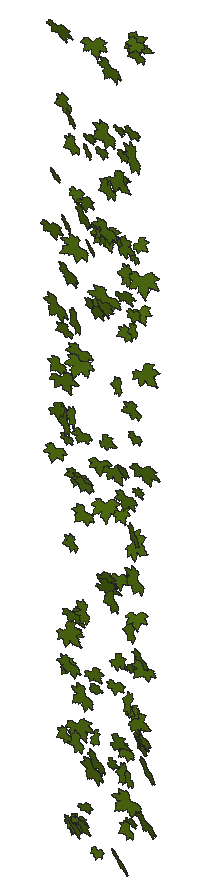
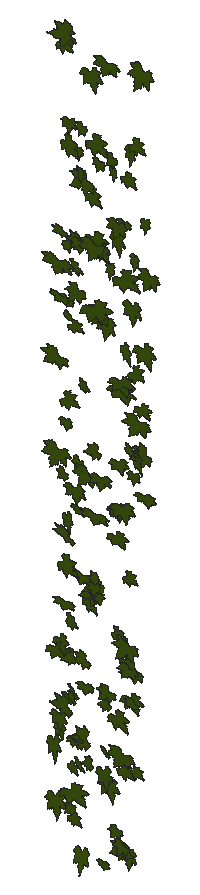
# SketchUp Ruby script. Lengths in inches.
U = 1.inch
M = Sketchup.active_model
def pt(a) = Geom::Point3d.new(a.map { |v| v * U })
def face(e, loops, mat)
  f = e.add_face(loops[0].map { |a| pt(a) })
  loops[1..].each { |l| e.add_face(l.map { |a| pt(a) }).erase! }
  f.material = f.back_material = mat if mat
  f
end
# faces: each face lists its corners as indices into pts; further lists are holes
def faces(e, pts, list, mat = nil) = list.each { |f| face(e, (f[0].is_a?(Array) ? f : [f]).map { |l| l.map { |i| pts[i] } }, mat) }
# xy, xz, yz: faces in a plane at the given z, y or x. An outline is a flat list of corners, or four numbers for a rectangle; further outlines are holes
def ring(l) = l.size == 4 ? [[l[0], l[1]], [l[2], l[1]], [l[2], l[3]], [l[0], l[3]]] : l.each_slice(2).to_a
def flat(e, list, mat, &to3) = list.each { |f| face(e, (f[0].is_a?(Array) ? f : [f]).map { |l| ring(l).map { |u, v| to3.(u, v) } }, mat) }
def xy(e, z, list, mat = nil) = flat(e, list, mat) { |x, y| [x, y, z] }
def xz(e, y, list, mat = nil) = flat(e, list, mat) { |x, z| [x, y, z] }
def yz(e, x, list, mat = nil) = flat(e, list, mat) { |y, z| [x, y, z] }
def lines(e, pts, list) = list.each { |a, b| e.add_line(pt(pts[a]), pt(pts[b])) }
# prism: a flat outline (further loops are holes) pulled along v
def prism(e, loops, v, mat = nil)
  f = face(e, loops, mat); d = Geom::Vector3d.new(v.map { |x| x * U })
  f.pushpull(f.normal.samedirection?(d) ? d.length : -d.length)
end
def box(e, o, s, mat = nil) = prism(e, [[o, [o[0] + s[0], o[1], o[2]], [o[0] + s[0], o[1] + s[1], o[2]], [o[0], o[1] + s[1], o[2]]]], [0, 0, s[2]], mat)
def at(x, y, z, deg = 0) = Geom::Transformation.translation(pt([x, y, z])) * Geom::Transformation.rotation(ORIGIN, Z_AXIS, deg.degrees)
def axes(o, x, y, z) = Geom::Transformation.new([*x, 0, *y, 0, *z, 0, *pt(o).to_a, 1])
def part(name) = M.definitions.add(name)
# library, detail: a bought-in or finely detailed component or shape, given as its bounding box
def library(name, o, s) = part(name).tap { |d| box(d.entities, o, s) }
def detail(e, o, s) = box(e.add_group.entities, o, s)
def put(e, d, t, mat = nil) = e.add_instance(d, t).tap { |i| i.material = mat if mat }
def group(e, t, mat = nil) = e.add_group.tap { |g| g.transformation = t; g.material = mat if mat }.entities
root = M.entities
M.materials.add("[Vegetation Blur 03]").color = [83, 114, 18]
c1 = part("ivy")
xy(c1.entities,0,[[0.782,0,0.786,0,0.787,0.005,0.789,0.009,0.821,0.072,0.875,0.147,1.001,0.272,1.073,0.331,1.137,0.363,1.178,0.379,1.223,0.384,1.272,0.383,1.311,0.374,1.36,0.355,1.399,0.334,1.491,0.285,1.541,0.244,1.583,0.199,1.617,0.15,1.64,0.128,1.662,0.115,1.717,0.105,1.745,0.093,1.784,0.054,1.819,0.057,1.854,0.064,1.882,0.075,1.896,0.074,1.91,0.071,1.937,0.063,1.964,0.053,1.99,0.038,2.016,0.015,2.034,0.002,2.04,0,2.038,0.003,2.036,0.007,2.033,0.038,2.036,0.068,2.045,0.1,2.055,0.116,2.064,0.123,2.077,0.129,2.088,0.129,2.106,0.132,2.118,0.13,2.179,0.132,2.207,0.133,2.225,0.133,2.242,0.138,2.22,0.162,2.207,0.186,2.206,0.213,2.212,0.236,2.228,0.262,2.247,0.274,2.298,0.283,2.355,0.294,2.37,0.296,2.376,0.295,2.377,0.3,2.377,0.303,2.385,0.329,2.411,0.37,2.426,0.392,2.449,0.407,2.511,0.426,2.561,0.444,2.619,0.466,2.589,0.469,2.561,0.476,2.501,0.5,2.449,0.516,2.424,0.523,2.401,0.535,2.377,0.556,2.372,0.568,2.36,0.575,2.268,0.586,2.225,0.592,2.207,0.599,2.194,0.61,2.143,0.65,2.13,0.664,2.122,0.682,2.123,0.7,2.13,0.719,2.148,0.75,2.17,0.781,2.195,0.807,2.221,0.828,2.284,0.874,2.291,0.88,2.288,0.887,2.276,0.9,2.267,0.916,2.265,0.933,2.273,0.967,2.292,1.002,2.313,1.03,2.334,1.054,2.348,1.067,2.358,1.074,2.363,1.076,2.362,1.081,2.35,1.094,2.347,1.11,2.35,1.143,2.359,1.18,2.385,1.254,2.415,1.324,2.448,1.393,2.45,1.4,2.446,1.398,2.44,1.394,2.427,1.383,2.402,1.36,2.376,1.339,2.345,1.324,2.305,1.309,2.282,1.303,2.273,1.306,2.245,1.294,2.212,1.287,2.187,1.291,2.163,1.301,2.142,1.316,2.134,1.327,2.124,1.325,2.09,1.292,2.053,1.259,2.014,1.234,1.973,1.215,1.954,1.21,1.931,1.208,1.909,1.212,1.893,1.22,1.879,1.233,1.872,1.248,1.867,1.281,1.864,1.319,1.821,1.258,1.773,1.197,1.726,1.141,1.698,1.121,1.679,1.116,1.666,1.117,1.647,1.122,1.632,1.129,1.62,1.141,1.617,1.154,1.617,1.219,1.621,1.254,1.623,1.268,1.623,1.281,1.618,1.314,1.606,1.346,1.603,1.375,1.607,1.403,1.603,1.467,1.599,1.499,1.605,1.525,1.614,1.552,1.629,1.577,1.635,1.589,1.629,1.587,1.618,1.582,1.596,1.566,1.581,1.556,1.568,1.552,1.557,1.55,1.545,1.553,1.531,1.562,1.522,1.572,1.504,1.591,1.486,1.611,1.474,1.631,1.457,1.666,1.455,1.684,1.457,1.698,1.452,1.715,1.444,1.728,1.424,1.754,1.419,1.772,1.423,1.786,1.434,1.819,1.444,1.848,1.446,1.855,1.44,1.861,1.43,1.867,1.386,1.904,1.349,1.948,1.326,1.973,1.31,1.995,1.288,2.048,1.284,2.153,1.287,2.254,1.284,2.255,1.282,2.253,1.278,2.247,1.274,2.237,1.266,2.216,1.226,2.125,1.208,2.076,1.184,2.033,1.155,1.984,1.135,1.942,1.111,1.899,1.083,1.861,1.053,1.85,1.059,1.83,1.061,1.809,1.056,1.79,1.049,1.767,1.04,1.749,1.018,1.733,0.994,1.726,0.942,1.734,0.95,1.6875,0.944,1.645,0.932,1.608,0.911,1.585,0.881,1.58,0.854,1.582,0.828,1.588,0.785,1.618,0.773,1.625,0.775,1.614,0.779,1.598,0.796,1.502,0.818,1.402,0.861,1.283,0.882,1.224,0.894,1.174,0.892,1.148,0.886,1.123,0.881,1.107,0.872,1.099,0.849,1.094,0.818,1.092,0.789,1.098,0.762,1.107,0.753,1.113,0.721,1.139,0.698,1.163,0.678,1.194,0.665,1.224,0.628,1.28,0.612,1.312,0.606,1.327,0.606,1.314,0.599,1.282,0.594,1.267,0.581,1.256,0.544,1.245,0.512,1.244,0.473,1.249,0.444,1.256,0.382,1.288,0.339,1.306,0.324,1.316,0.317,1.324,0.309,1.326,0.27,1.314,0.227,1.313,0.185,1.3125,0.152,1.317,0.122,1.328,0.092,1.345,0.073,1.353,0.079,1.338,0.092,1.308,0.117,1.249,0.13,1.215,0.139,1.164,0.147,1.148,0.157,1.136,0.163,1.122,0.174,1.086,0.177,1.067,0.182,1.054,0.186,1.043,0.191,1.038,0.211,1.028,0.237,1.005,0.25,0.974,0.253,0.96,0.25,0.944,0.242,0.914,0.243,0.906,0.249,0.902,0.26,0.894,0.289,0.88,0.307,0.873,0.322,0.862,0.364,0.799,0.403,0.738,0.431,0.709,0.439,0.691,0.441,0.678,0.4375,0.66,0.428,0.645,0.394,0.623,0.303,0.594,0.255,0.581,0.214,0.577,0.179,0.573,0.173,0.568,0.175,0.561,0.167,0.55,0.141,0.523,0.113,0.503,0.077,0.49,0.045,0.486,0.026,0.485,0.019,0.486,0.011,0.483,0,0.471,0.014,0.467,0.044,0.455,0.058,0.447,0.07,0.438,0.097,0.411,0.125,0.394,0.158,0.377,0.174,0.366,0.182,0.359,0.185,0.361,0.242,0.331,0.253,0.316,0.258,0.303,0.262,0.283,0.274,0.278,0.308,0.274,0.341,0.252,0.366,0.226,0.366,0.222,0.37,0.22,0.38,0.221,0.395,0.221,0.425,0.216,0.45,0.207,0.465,0.192,0.473,0.178,0.484,0.15,0.489,0.116,0.483,0.089,0.468,0.058,0.45,0.035,0.435,0.018,0.429,0.011,0.434,0.012,0.438,0.014,0.469,0.019,0.542,0.016,0.581,0.015,0.612,0.027,0.68,0.055,0.696,0.057,0.712,0.052,0.73,0.045,0.741,0.036,0.766,0.014]])
put(root,c1,axes([25.61,173.2,133.48],[0.51847,-0.08238,0.09913],[0.12469,0.09368,-0.42215],[-0.02842,-1.09178,-0.0437]),"[Vegetation Blur 03]")
put(root,c1,axes([26.27,173.2,136.41],[0.29856,-0.10941,-0.11062],[-0.12269,0.1536,-0.24445],[-0.0784,-0.65702,-0.03873]),"[Vegetation Blur 03]")
put(root,c1,axes([26.22,173.2,130.02],[0.54012,-0.12372,-0.29412],[-0.3556,0.12595,-0.44329],[-0.0839,-1.33021,-0.01462]),"[Vegetation Blur 03]")
put(root,c1,axes([26.06,173.2,122.15],[0.44019,0.01869,-0.05575],[-0.06711,-0.08998,-0.3577],[0.01564,-0.91223,0.03414]),"[Vegetation Blur 03]")
put(root,c1,axes([26.51,173.2,126.82],[0.32974,-0.02071,-0.22461],[-0.27537,-0.01528,-0.26905],[-0.00296,-0.88368,0.00992]),"[Vegetation Blur 03]")
put(root,c1,axes([27.09,173.2,128.67],[0.16409,0.0678,-0.30247],[-0.37206,0.03564,-0.13319],[-0.00256,-0.83328,-0.0303]),"[Vegetation Blur 03]")
put(root,c1,axes([26.08,173.2,123.74],[0.26787,-0.06927,0.33281],[0.40897,0.07748,-0.21671],[0.01312,-1.00101,-0.0398]),"[Vegetation Blur 03]")
put(root,c1,axes([25.9375,173.2,143.96],[0.62307,-0.149,0.09151],[0.12235,0.19755,-0.50432],[-0.05332,-1.28769,-0.08796]),"[Vegetation Blur 03]")
put(root,c1,axes([27.1,173.2,140.49],[0.19509,-0.01615,-0.32843],[-0.40182,0.04546,-0.15934],[-0.0233,-0.91916,-0.00211]),"[Vegetation Blur 03]")
put(root,c1,axes([27.05,173.2,124.49],[0.3874,-0.28987,-0.42046],[-0.49062,0.32448,-0.33628],[-0.21109,-1.28615,0.00992]),"[Vegetation Blur 03]")
put(root,c1,axes([27.08,173.2,107.82],[0.20749,-0.03484,-0.23563],[-0.28917,-0.01288,-0.16931],[-0.00479,-0.73151,0.0142]),"[Vegetation Blur 03]")
put(root,c1,axes([26.09,173.2,125.65],[0.54429,0.0275,0.19656],[0.23996,0.06284,-0.44397],[0.02457,-1.22318,-0.01839]),"[Vegetation Blur 03]")
put(root,c1,axes([26.86,173.2,122.97],[0.32248,-0.05987,-0.04087],[-0.04757,0.05862,-0.26354],[-0.03303,-0.669,-0.01944]),"[Vegetation Blur 03]")
put(root,c1,axes([26.92,173.2,134.23],[0.34481,-0.20074,-0.10306],[-0.10927,0.15385,-0.29065],[-0.11628,-0.7398,-0.03248]),"[Vegetation Blur 03]")
put(root,c1,axes([26.96,173.2,111.59],[0.47072,-0.03676,-0.23219],[-0.28418,0.02801,-0.38445],[-0.02233,-1.13149,-0.00197]),"[Vegetation Blur 03]")
put(root,c1,axes([27.53,173.2,117.86],[0.16539,-0.02327,-0.29289],[-0.35869,0.02592,-0.13523],[-0.01618,-0.81273,0.00407]),"[Vegetation Blur 03]")
put(root,c1,axes([26.79,173.2,131.81],[0.56634,-0.19077,-0.13861],[-0.15859,0.16167,-0.4666],[-0.11086,-1.2059,-0.04063]),"[Vegetation Blur 03]")
put(root,c1,axes([26.82,173.2,110.78],[0.17104,0.07406,0.23051],[0.28468,-0.03259,-0.13906],[0.00499,-0.6787,0.03183]),"[Vegetation Blur 03]")
put(root,c1,axes([27.67,173.2,124.4375],[0.12105,-0.13191,-0.28197],[-0.3442,0.10689,-0.10629],[-0.07075,-0.74572,0.03464]),"[Vegetation Blur 03]")
put(root,c1,axes([27.51,173.2,138.55],[0.26106,-0.06742,-0.29363],[-0.35973,0.03582,-0.21432],[-0.03335,-0.91402,0.01326]),"[Vegetation Blur 03]")
put(root,c1,axes([27.14,173.2,139.82],[0.38591,-0.21569,-0.14541],[-0.15737,0.19687,-0.32414],[-0.13402,-0.85224,-0.03808]),"[Vegetation Blur 03]")
put(root,c1,axes([26.49,173.2,112.35],[0.3582,0.03063,0.42978],[0.52659,-0.05959,-0.29166],[-0.01559,-1.30923,0.02333]),"[Vegetation Blur 03]")
put(root,c1,axes([26.84,173.2,112.62],[0.36162,0.06548,0.17991],[0.22033,0.0215,-0.29621],[0.03262,-0.87124,0.00621]),"[Vegetation Blur 03]")
put(root,c1,axes([27.63,173.2,133.49],[0.37878,0.01189,-0.41383],[-0.50562,-0.09055,-0.30867],[0.03871,-1.29927,0.01773]),"[Vegetation Blur 03]")
put(root,c1,axes([27.08,173.2,103.34],[0.50401,-0.18357,-0.11952],[-0.1351,0.15116,-0.41597],[-0.10561,-1.06941,-0.03828]),"[Vegetation Blur 03]")
put(root,c1,axes([27.61,173.2,129.625],[0.34504,-0.21965,-0.31495],[-0.37042,0.22285,-0.29474],[-0.152,-1.04167,0.00335]),"[Vegetation Blur 03]")
put(root,c1,axes([27.85,173.2,107.85],[0.21313,-0.07118,-0.35531],[-0.43534,0.04461,-0.17534],[-0.03471,-0.99647,0.01753]),"[Vegetation Blur 03]")
put(root,c1,axes([27.26,173.2,121.31],[0.48743,0.04761,-0.1367],[-0.16843,0.04371,-0.39762],[0.01495,-1.05971,-0.02254]),"[Vegetation Blur 03]")
put(root,c1,axes([26.79,173.2,113.73],[0.50143,-0.04661,0.23263],[0.28578,0.12116,-0.40648],[0.00953,-1.18071,-0.05089]),"[Vegetation Blur 03]")
put(root,c1,axes([27.12,173.2,102.72],[0.18512,0.00647,0.33943],[0.41367,-0.0999,-0.14998],[-0.04308,-0.93144,0.01844]),"[Vegetation Blur 03]")
put(root,c1,axes([27.39,173.2,135.79],[0.32765,-0.02489,0.01881],[0.02157,-0.07508,-0.26601],[-0.01455,-0.67173,0.02903]),"[Vegetation Blur 03]")
put(root,c1,axes([27.42,173.2,127.85],[0.50815,0.02983,-0.17456],[-0.21367,-0.02159,-0.41487],[0.01743,-1.13431,0.00331]),"[Vegetation Blur 03]")
put(root,c1,axes([27.4,173.2,127.3],[0.55742,0.02012,-0.13001],[-0.15728,-0.13301,-0.4524],[0.0271,-1.18554,0.04855]),"[Vegetation Blur 03]")
put(root,c1,axes([27.63,173.2,123.5],[0.38921,0.02788,-0.11804],[-0.14492,0.01541,-0.31769],[0.01009,-0.85429,-0.00958]),"[Vegetation Blur 03]")
put(root,c1,axes([27.62,173.2,121.16],[0.40951,0.01971,-0.10583],[-0.13003,0.06915,-0.33309],[-0.00105,-0.88123,-0.0285]),"[Vegetation Blur 03]")
put(root,c1,axes([27.39,173.2,103.37],[0.37849,-0.06704,0.09137],[0.11442,0.06293,-0.30843],[-0.02244,-0.80977,-0.03153]),"[Vegetation Blur 03]")
put(root,c1,axes([27.02,173.2,108.03],[0.53376,0.03726,0.21952],[0.269,0.00727,-0.43585],[0.01776,-1.22992,0.00407]),"[Vegetation Blur 03]")
put(root,c1,axes([27.98,173.2,110.45],[0.42826,-0.11256,-0.35023],[-0.42906,0.04831,-0.35189],[-0.05529,-1.24664,0.01798]),"[Vegetation Blur 03]")
put(root,c1,axes([28.31,173.2,114.72],[0.19822,-0.13225,-0.36337],[-0.44645,0.06503,-0.16594],[-0.0552,-1.0008,0.03723]),"[Vegetation Blur 03]")
put(root,c1,axes([27.91,173.2,119.69],[0.40363,-0.02669,-0.22372],[-0.27442,-0.04788,-0.32887],[0.00236,-1.00289,0.02165]),"[Vegetation Blur 03]")
put(root,c1,axes([27.85,173.2,121.06],[0.38167,-0.01698,-0.15187],[-0.18516,0.0606,-0.31101],[-0.02031,-0.87168,-0.01866]),"[Vegetation Blur 03]")
put(root,c1,axes([27.84,173.2,135.18],[0.47471,-0.2198,-0.23723],[-0.27334,0.21714,-0.39597],[-0.14555,-1.12467,-0.03009]),"[Vegetation Blur 03]")
put(root,c1,axes([27.5625,173.2,135.6],[0.49002,-0.06773,0.03255],[0.04203,0.06603,-0.39982],[-0.03013,-1.00954,-0.02833]),"[Vegetation Blur 03]")
put(root,c1,axes([27.77,173.2,104.02],[0.2717,-0.01326,0.11926],[0.14597,0.06528,-0.22036],[0.00938,-0.63148,-0.02528]),"[Vegetation Blur 03]")
put(root,c1,axes([27.55,173.2,102.9],[0.29257,-0.13243,0.26003],[0.3239,0.04481,-0.23915],[-0.02726,-0.88901,-0.05079]),"[Vegetation Blur 03]")
put(root,c1,axes([28.23,173.2,138.33],[0.2858,-0.16556,-0.09391],[-0.1058,0.0991,-0.24194],[-0.0923,-0.62621,-0.01346]),"[Vegetation Blur 03]")
put(root,c1,axes([28.31,173.2,133.39],[0.30779,-0.16022,-0.12096],[-0.12595,0.19898,-0.2549],[-0.11031,-0.67423,-0.04648]),"[Vegetation Blur 03]")
put(root,c1,axes([28.1,173.2,138.75],[0.27595,-0.07999,0.10883],[0.13684,0.05207,-0.2251],[-0.02378,-0.62852,-0.0325]),"[Vegetation Blur 03]")
put(root,c1,axes([28.26,173.2,106.78],[0.5571,-0.15804,-0.2532],[-0.30286,0.14883,-0.45846],[-0.10211,-1.30372,-0.02164]),"[Vegetation Blur 03]")
put(root,c1,axes([28.12,173.2,110.93],[0.31712,0.01449,0.22059],[0.2693,0.0595,-0.25849],[0.0241,-0.85537,-0.01424]),"[Vegetation Blur 03]")
put(root,c1,axes([27.97,173.2,143.6875],[0.52799,0.03971,0.1403],[0.17249,-0.03446,-0.43082],[0.01316,-1.14211,0.01788]),"[Vegetation Blur 03]")
put(root,c1,axes([28.26,173.2,130.47],[0.55471,-0.15442,-0.09413],[-0.10485,0.16405,-0.45388],[-0.08911,-1.1543,-0.05191]),"[Vegetation Blur 03]")
put(root,c1,axes([28.57,173.2,107.23],[0.48731,-0.17978,-0.24983],[-0.29064,0.21865,-0.40235],[-0.12987,-1.16387,-0.037]),"[Vegetation Blur 03]")
put(root,c1,axes([28.97,173.2,134.43],[0.27575,-0.07071,-0.32237],[-0.38727,0.16418,-0.22631],[-0.08498,-0.9776,-0.01469]),"[Vegetation Blur 03]")
put(root,c1,axes([28.52,173.2,110.13],[0.08923,-0.0651,0.22881],[0.28147,0.0622,-0.07033],[0.01942,-0.60224,-0.032]),"[Vegetation Blur 03]")
put(root,c1,axes([28.55,173.2,107.58],[0.08406,0.07505,0.23958],[0.28752,-0.16835,-0.0589],[-0.06954,-0.60538,0.04608]),"[Vegetation Blur 03]")
put(root,c1,axes([28.66,173.2,102.17],[0.29298,-0.03076,-0.00517],[-0.00747,-0.046,-0.2387],[-0.01442,-0.60127,0.01853]),"[Vegetation Blur 03]")
put(root,c1,axes([28.49,173.2,122.21],[0.45127,0.0715,0.00789],[0.01018,-0.0128,-0.36935],[0.0346,-0.92876,0.0057]),"[Vegetation Blur 03]")
put(root,c1,axes([28.98,173.2,131.38],[0.53259,0.07407,-0.33493],[-0.4092,-0.06459,-0.43565],[0.04766,-1.38209,0.00241]),"[Vegetation Blur 03]")
put(root,c1,axes([29.35,173.2,139.9375],[0.36403,-0.06267,-0.40957],[-0.5016,0.04126,-0.29795],[-0.03412,-1.27511,0.01049]),"[Vegetation Blur 03]")
put(root,c1,axes([28.84,173.2,138.38],[0.31483,-0.06922,0.03461],[0.04453,0.03834,-0.25772],[-0.03078,-0.65259,-0.01881]),"[Vegetation Blur 03]")
put(root,c1,axes([29.11,173.2,134.875],[0.46325,-0.03451,-0.29794],[-0.36488,0.02419,-0.37832],[-0.02045,-1.21347,0.00093]),"[Vegetation Blur 03]")
put(root,c1,axes([29.59,173.2,137.03],[0.26205,-0.06963,-0.34462],[-0.42004,0.08964,-0.2156],[-0.05487,-1.01871,0.00458]),"[Vegetation Blur 03]")
put(root,c1,axes([29.12,173.2,116.43],[0.29824,-0.02143,-0.02343],[-0.02665,0.10046,-0.24043],[-0.01491,-0.60833,-0.03888]),"[Vegetation Blur 03]")
put(root,c1,axes([28.47,173.2,134.03],[0.60611,0.08882,0.16972],[0.20851,-0.00255,-0.49577],[0.04043,-1.31863,0.01239]),"[Vegetation Blur 03]")
put(root,c1,axes([28.64,173.2,120.07],[0.5345,0.11261,0.12686],[0.16236,-0.17388,-0.43135],[0.02823,-1.13219,0.07887]),"[Vegetation Blur 03]")
put(root,c1,axes([28.8125,173.2,130.49],[0.44672,-0.11391,0.09884],[0.12385,0.0351,-0.3665],[-0.0489,-0.9518,-0.02535]),"[Vegetation Blur 03]")
put(root,c1,axes([29.03,173.2,122.99],[0.12471,-0.00455,0.29508],[0.36083,0.05141,-0.10146],[0.0229,-0.78534,-0.00835]),"[Vegetation Blur 03]")
put(root,c1,axes([29.1875,173.2,143.26],[0.56003,-0.11483,-0.22477],[-0.26984,0.13286,-0.4585],[-0.07841,-1.27735,-0.02748]),"[Vegetation Blur 03]")
put(root,c1,axes([28.82,173.2,116.17],[0.35675,-0.1356,0.28151],[0.35114,0.1247,-0.28695],[-0.00453,-1.0135,-0.07297]),"[Vegetation Blur 03]")
put(root,c1,axes([29.75,173.2,115.94],[0.31943,-0.14813,-0.35105],[-0.42397,0.15166,-0.26703],[-0.10221,-1.09204,0.01053]),"[Vegetation Blur 03]")
put(root,c1,axes([28.84,173.2,115.58],[0.27593,-0.17427,0.39331],[0.48854,0.16147,-0.21704],[0.02723,-1.13128,-0.09157]),"[Vegetation Blur 03]")
put(root,c1,axes([29.56,173.2,106.65],[0.09053,-0.05831,0.23092],[0.28382,-0.01925,-0.07488],[-0.01758,-0.61103,-0.01968]),"[Vegetation Blur 03]")
put(root,c1,axes([29.54,173.2,111.08],[0.35798,0.03491,0.00358],[0.00487,-0.0205,-0.29237],[0.01684,-0.73641,0.00831]),"[Vegetation Blur 03]")
put(root,c1,axes([29.14,173.2,121.9],[0.48195,0.00963,0.21143],[0.25864,0.04977,-0.39304],[0.01557,-1.12486,-0.01558]),"[Vegetation Blur 03]")
put(root,c1,axes([30.34,173.2,126.88],[0.08976,-0.09939,-0.28739],[-0.34963,0.10974,-0.07871],[-0.06393,-0.7397,0.02694]),"[Vegetation Blur 03]")
put(root,c1,axes([29.76,173.2,102.52],[0.54071,-0.2448,-0.19934],[-0.20803,0.34691,-0.44288],[-0.17473,-1.17061,-0.08956]),"[Vegetation Blur 03]")
put(root,c1,axes([29.83,173.2,134.13],[0.37713,0.02521,-0.05482],[-0.06814,0.09104,-0.30568],[0.00422,-0.78299,-0.03731]),"[Vegetation Blur 03]")
put(root,c1,axes([29.66,173.2,116.58],[0.38704,0.02073,0.09682],[0.11906,-0.06304,-0.31489],[0.00062,-0.83064,0.02631]),"[Vegetation Blur 03]")
put(root,c1,axes([29.86,173.2,139.86],[0.29162,-0.09248,0.04712],[0.06325,0.07335,-0.23812],[-0.03677,-0.60733,-0.03593]),"[Vegetation Blur 03]")
put(root,c1,axes([29.625,173.2,111.95],[0.20869,-0.00294,0.30527],[0.37402,-0.00987,-0.17032],[-0.00489,-0.88135,0.00089]),"[Vegetation Blur 03]")
put(root,c1,axes([29.34,173.2,136.79],[0.38841,-0.03974,0.39058],[0.47889,0.01108,-0.31703],[-0.00798,-1.26829,-0.01501]),"[Vegetation Blur 03]")
put(root,c1,axes([30.14,173.2,137.65],[0.29613,-0.07388,-0.10232],[-0.12287,0.05638,-0.24327],[-0.04369,-0.65932,-0.00934]),"[Vegetation Blur 03]")
put(root,c1,axes([30.625,173.2,107.11],[0.14128,-0.20319,-0.29587],[-0.36071,0.14973,-0.1309],[-0.10517,-0.78653,0.05152]),"[Vegetation Blur 03]")
put(root,c1,axes([29.74,173.2,107.61],[0.11289,-0.08937,0.40816],[0.50197,0.01041,-0.09212],[-0.00461,-1.05497,-0.03549]),"[Vegetation Blur 03]")
put(root,c1,axes([30.17,173.2,138.74],[0.29319,-0.08212,-0.05398],[-0.06371,0.04494,-0.24127],[-0.04367,-0.61685,-0.01039]),"[Vegetation Blur 03]")
put(root,c1,axes([29.86,173.2,119.81],[0.27283,0.0757,0.1916],[0.23721,-0.13013,-0.2169],[-0.01401,-0.72914,0.0586]),"[Vegetation Blur 03]")
put(root,c1,axes([30.64,173.2,129.78],[0.19574,-0.01438,-0.25163],[-0.30815,-0.03945,-0.1593],[0.01245,-0.75048,0.0132]),"[Vegetation Blur 03]")
put(root,c1,axes([30.41,173.2,105.83],[0.47968,0.02946,-0.35016],[-0.4281,-0.06549,-0.39149],[0.03188,-1.32271,0.01158]),"[Vegetation Blur 03]")
put(root,c1,axes([30.91,173.2,132.9],[0.09556,-0.13792,-0.34176],[-0.41905,0.10501,-0.08471],[-0.06516,-0.87761,0.04357]),"[Vegetation Blur 03]")
put(root,c1,axes([30.05,173.2,122.375],[0.34163,-0.14558,0.05444],[0.07406,0.06471,-0.28235],[-0.063,-0.71335,-0.03672]),"[Vegetation Blur 03]")
put(root,c1,axes([30.51,173.2,108.26],[0.31122,-0.06083,-0.21678],[-0.26689,-0.02709,-0.25402],[-0.01391,-0.84152,0.02385]),"[Vegetation Blur 03]")
put(root,c1,axes([30.66,173.2,104.21],[0.24157,-0.07416,-0.2538],[-0.31175,0.01688,-0.19842],[-0.02861,-0.81014,0.0191]),"[Vegetation Blur 03]")
put(root,c1,axes([29.86,173.2,131.19],[0.40086,-0.0573,0.17483],[0.21594,0.13183,-0.32299],[0.00594,-0.92596,-0.0568]),"[Vegetation Blur 03]")
put(root,c1,axes([30.07,173.2,121.18],[0.52679,-0.06661,-0.07919],[-0.09633,0.02908,-0.43069],[-0.03439,-1.10187,-0.00658]),"[Vegetation Blur 03]")
put(root,c1,axes([31.05,173.2,110.77],[0.05013,-0.17245,-0.31461],[-0.38087,0.18721,-0.05657],[-0.1028,-0.77773,0.05615]),"[Vegetation Blur 03]")
put(root,c1,axes([30.75,173.2,106.8],[0.21308,-0.10262,-0.22404],[-0.27243,0.07685,-0.17812],[-0.0602,-0.71097,0.01308]),"[Vegetation Blur 03]")
put(root,c1,axes([31.07,173.2,114.47],[0.09612,-0.08439,-0.33414],[-0.40558,0.12635,-0.08273],[-0.06933,-0.85613,0.02072]),"[Vegetation Blur 03]")
put(root,c1,axes([30.16,173.2,133.32],[0.06821,0.02412,0.38984],[0.47536,-0.1037,-0.05439],[-0.04826,-0.98747,0.01524]),"[Vegetation Blur 03]")
put(root,c1,axes([31.08,173.2,125.97],[0.16222,0.03807,-0.33908],[-0.41557,-0.02093,-0.13279],[0.01621,-0.91758,-0.01104]),"[Vegetation Blur 03]")
put(root,c1,axes([31.03,173.2,139.36],[0.33503,-0.17484,-0.44401],[-0.53885,0.1655,-0.28108],[-0.11328,-1.30432,0.02385]),"[Vegetation Blur 03]")
put(root,c1,axes([30.55,173.2,140.1],[0.37183,-0.05449,-0.06268],[-0.07386,0.08152,-0.30299],[-0.03383,-0.77703,-0.02739]),"[Vegetation Blur 03]")
put(root,c1,axes([31.18,173.2,117.5],[0.29364,-0.08887,-0.43973],[-0.53794,0.07502,-0.24166],[-0.05272,-1.26047,0.01662]),"[Vegetation Blur 03]")
put(root,c1,axes([30.56,173.2,109.67],[0.05383,0.00628,0.24765],[0.29967,-0.10102,-0.04299],[-0.04781,-0.62607,0.00942]),"[Vegetation Blur 03]")
put(root,c1,axes([30.48,173.2,111.97],[0.19108,-0.09038,0.20852],[0.25839,0.11931,-0.14958],[0.021,-0.6456,-0.05683]),"[Vegetation Blur 03]")
put(root,c1,axes([30.95,173.2,133.79],[0.23501,-0.07019,-0.1629],[-0.19555,0.08472,-0.19365],[-0.05258,-0.62881,-0.00791]),"[Vegetation Blur 03]")
put(root,c1,axes([30.875,173.2,119.66],[0.37161,-0.21861,-0.25288],[-0.28876,0.23657,-0.31481],[-0.15463,-0.96714,-0.01984]),"[Vegetation Blur 03]")
put(root,c1,axes([30.51,173.2,104.28],[0.2775,-0.12673,0.11481],[0.14869,0.07236,-0.22682],[-0.03837,-0.63611,-0.04867]),"[Vegetation Blur 03]")
put(root,c1,axes([31.21,173.2,144.4],[0.21316,0.03069,-0.31446],[-0.38542,0.04396,-0.17335],[-0.01149,-0.90506,-0.01908]),"[Vegetation Blur 03]")
put(root,c1,axes([31.13,173.2,130.06],[0.16581,-0.12598,-0.20066],[-0.24842,0.03821,-0.1405],[-0.04988,-0.60905,0.03269]),"[Vegetation Blur 03]")
put(root,c1,axes([30.82,173.2,124.42],[0.33014,-0.06379,-0.05513],[-0.06679,0.02302,-0.2706],[-0.03261,-0.69306,-0.00391]),"[Vegetation Blur 03]")
put(root,c1,axes([30.7,173.2,109.71],[0.13106,0.04715,0.22271],[0.27208,-0.09295,-0.10355],[-0.03102,-0.61597,0.03267]),"[Vegetation Blur 03]")
put(root,c1,axes([30.68,173.2,130.65],[0.34203,-0.05341,0.04309],[0.05121,-0.04542,-0.27956],[-0.02898,-0.71072,0.01463]),"[Vegetation Blur 03]")
put(root,c1,axes([30.9,173.2,144.8125],[0.33694,0.0048,-0.1079],[-0.13035,-0.11296,-0.27192],[0.0222,-0.7362,0.04102]),"[Vegetation Blur 03]")
put(root,c1,axes([30.61,173.2,114.91],[0.41222,0.08825,0.09854],[0.12607,-0.1297,-0.333],[0.02291,-0.87434,0.05934]),"[Vegetation Blur 03]")
put(root,c1,axes([30.51,173.2,117.91],[0.09143,0.21564,0.47102],[0.58317,-0.16267,-0.06368],[-0.06308,-1.19139,0.09395]),"[Vegetation Blur 03]")
put(root,c1,axes([31.2,173.2,113.27],[0.3587,-0.08547,-0.26789],[-0.31864,0.17898,-0.29317],[-0.08908,-0.98439,-0.03004]),"[Vegetation Blur 03]")
put(root,c1,axes([31.28,173.2,108.8],[0.31159,-0.10577,-0.25159],[-0.29051,0.23223,-0.255],[-0.11522,-0.87155,-0.03742]),"[Vegetation Blur 03]")
put(root,c1,axes([30.5,173.2,143.86],[0.15219,-0.0035,0.49259],[0.60198,0.09401,-0.12377],[0.04388,-1.27745,-0.01046]),"[Vegetation Blur 03]")
put(root,c1,axes([30.96,173.2,121.4],[0.23912,-0.07387,0.13682],[0.16931,0.00875,-0.19635],[-0.02693,-0.60087,-0.01968]),"[Vegetation Blur 03]")
put(root,c1,axes([30.72,173.2,108.95],[0.10403,0.04174,0.45584],[0.55849,-0.05312,-0.08413],[-0.02168,-1.16792,0.02012]),"[Vegetation Blur 03]")
put(root,c1,axes([31.27,173.2,112.82],[0.41939,0.05909,-0.24373],[-0.29711,-0.06483,-0.343],[0.04165,-1.05748,0.00741]),"[Vegetation Blur 03]")
put(root,c1,axes([30.95,173.2,133.9],[0.15956,0.10306,0.24419],[0.30313,-0.02658,-0.13017],[0.01203,-0.69728,0.04105]),"[Vegetation Blur 03]")
put(root,c1,axes([31.16,173.2,109.1875],[0.45644,-0.12973,-0.15733],[-0.18474,0.13729,-0.3748],[-0.08372,-1.01031,-0.03073]),"[Vegetation Blur 03]")
put(root,c1,axes([30.87,173.2,130.54],[0.32504,0.10399,0.20827],[0.26014,-0.12611,-0.26052],[0.00118,-0.84097,0.06482]),"[Vegetation Blur 03]")
put(root,c1,axes([31.22,173.2,105.05],[0.5663,-0.16171,-0.26651],[-0.30497,0.30432,-0.46069],[-0.14072,-1.31032,-0.0741]),"[Vegetation Blur 03]")
put(root,c1,axes([30.66,173.2,132.52],[0.63449,0.08244,0.15008],[0.18708,-0.13099,-0.51549],[0.02055,-1.35306,0.05905]),"[Vegetation Blur 03]")
put(root,c1,axes([30.76,173.2,122.7],[0.61927,-0.03223,0.11526],[0.14207,0.12094,-0.50313],[-0.00213,-1.30144,-0.04961]),"[Vegetation Blur 03]")
put(root,c1,axes([31.5,173.2,107.85],[0.48214,-0.22782,-0.28181],[-0.31501,0.32234,-0.39997],[-0.17959,-1.177,-0.05499]),"[Vegetation Blur 03]")
put(root,c1,axes([30.82,173.2,127.27],[0.38223,0.09975,0.36551],[0.44923,0.00523,-0.31313],[0.03341,-1.2116,0.02874]),"[Vegetation Blur 03]")
